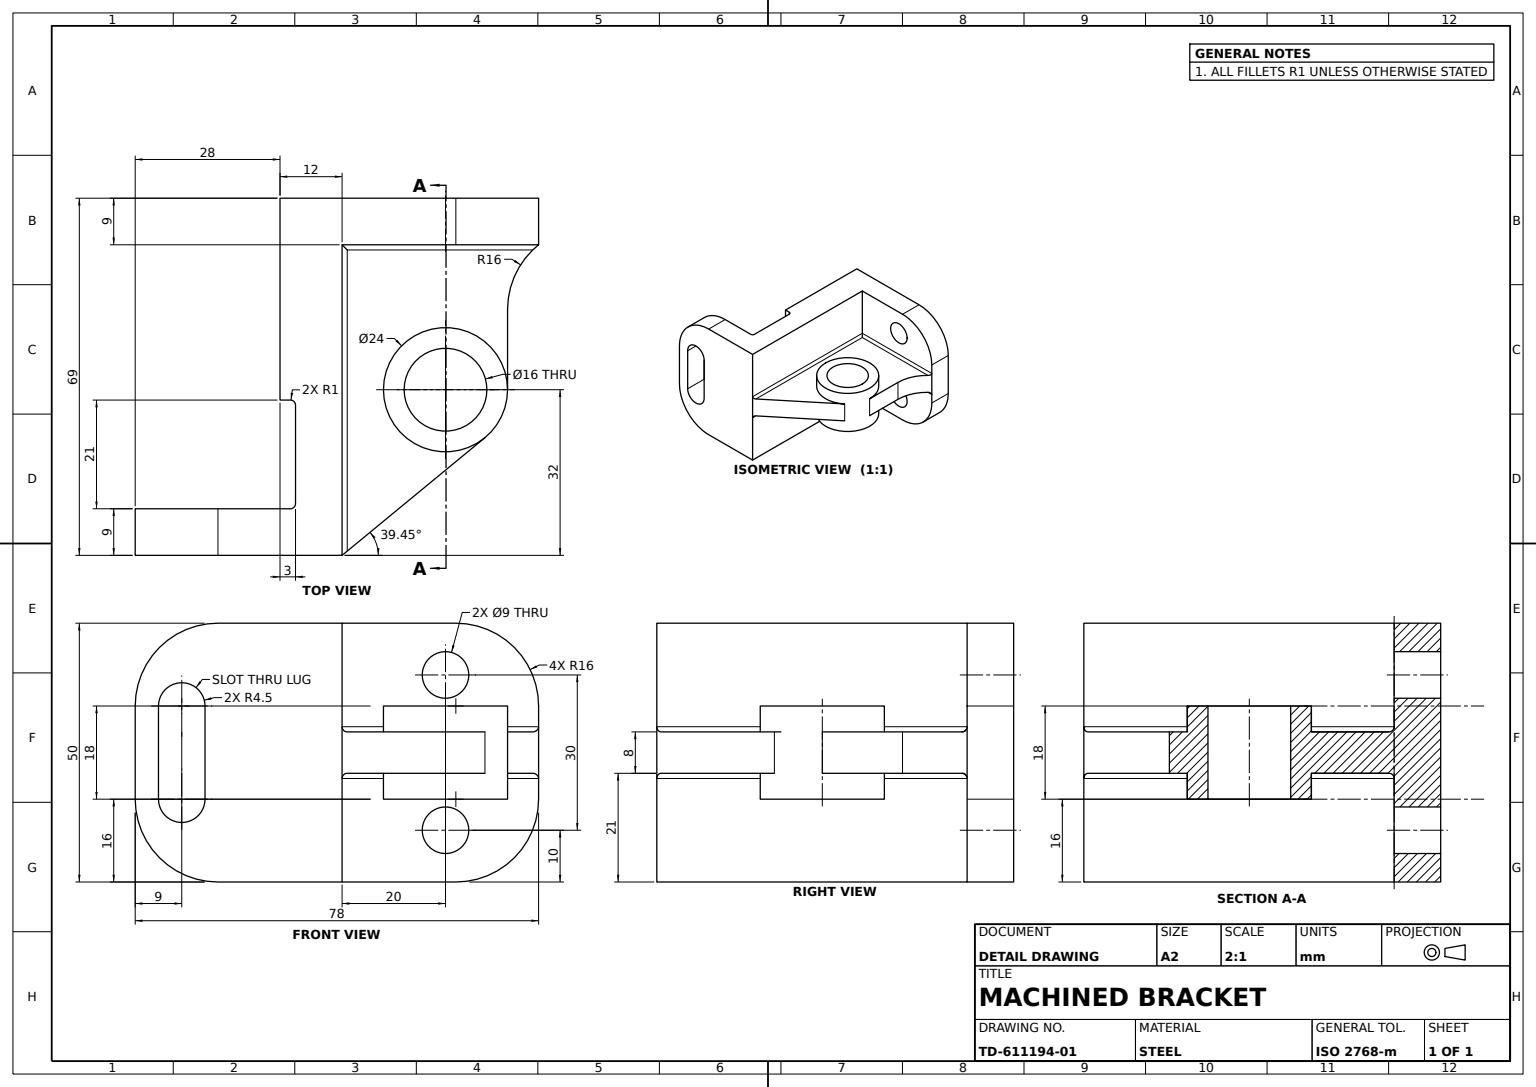
ISO-10303-21;
HEADER;
FILE_DESCRIPTION((''),'2;1');
FILE_NAME('','',(''),(''),'','','');
FILE_SCHEMA(('AUTOMOTIVE_DESIGN'));
ENDSEC;
DATA;
#1=APPLICATION_CONTEXT('');
#2=PRODUCT_CONTEXT('',#1,'mechanical');
#3=PRODUCT('','','',(#2));
#4=PRODUCT_DEFINITION_FORMATION('','',#3);
#5=PRODUCT_DEFINITION_CONTEXT('',#1,'design');
#6=PRODUCT_DEFINITION('','',#4,#5);
#7=PRODUCT_DEFINITION_SHAPE('','',#6);
#8=(LENGTH_UNIT()NAMED_UNIT(*)SI_UNIT(.MILLI.,.METRE.));
#9=(NAMED_UNIT(*)PLANE_ANGLE_UNIT()SI_UNIT($,.RADIAN.));
#10=(NAMED_UNIT(*)SI_UNIT($,.STERADIAN.)SOLID_ANGLE_UNIT());
#11=UNCERTAINTY_MEASURE_WITH_UNIT(LENGTH_MEASURE(1.E-05),#8,'distance_accuracy_value','');
#12=(GEOMETRIC_REPRESENTATION_CONTEXT(3)GLOBAL_UNCERTAINTY_ASSIGNED_CONTEXT((#11))GLOBAL_UNIT_ASSIGNED_CONTEXT((#8,#9,#10))REPRESENTATION_CONTEXT('',''));
#13=CARTESIAN_POINT('',(11.765801,-4.,-27.625282));
#14=VERTEX_POINT('',#13);
#15=CARTESIAN_POINT('',(33.677051,-4.,-1.));
#16=VERTEX_POINT('',#15);
#17=CARTESIAN_POINT('',(34.500404,-4.,0.000491));
#18=DIRECTION('',(0.635440172,0.,0.772150107));
#19=VECTOR('',#18,1000.);
#20=LINE('',#17,#19);
#21=EDGE_CURVE('',#14,#16,#20,.T.);
#22=ORIENTED_EDGE('',*,*,#21,.F.);
#23=CARTESIAN_POINT('',(11.765801,4.,-27.625282));
#24=VERTEX_POINT('',#23);
#25=CARTESIAN_POINT('',(11.765801,-14.,-27.625282));
#26=DIRECTION('',(0.,1.,0.));
#27=VECTOR('',#26,1000.);
#28=LINE('',#25,#27);
#29=EDGE_CURVE('',#14,#24,#28,.T.);
#30=ORIENTED_EDGE('',*,*,#29,.T.);
#31=CARTESIAN_POINT('',(33.677051,4.,-1.));
#32=VERTEX_POINT('',#31);
#33=CARTESIAN_POINT('',(34.5,4.,0.));
#34=LINE('',#33,#19);
#35=EDGE_CURVE('',#24,#32,#34,.T.);
#36=ORIENTED_EDGE('',*,*,#35,.T.);
#37=CARTESIAN_POINT('',(34.5,5.,0.));
#38=VERTEX_POINT('',#37);
#39=CARTESIAN_POINT('',(34.159123,4.,-0.414214));
#40=CARTESIAN_POINT('',(34.5,4.414214,0.));
#41=(BOUNDED_CURVE()B_SPLINE_CURVE(3,(#31,#39,#40,#37),.UNSPECIFIED.,.F.,.T.)B_SPLINE_CURVE_WITH_KNOTS((4,4),(1.570796327,3.141592654),.UNSPECIFIED.)CURVE()GEOMETRIC_REPRESENTATION_ITEM()RATIONAL_B_SPLINE_CURVE((1.,0.804737854,0.804737854,1.))REPRESENTATION_ITEM(''));
#42=EDGE_CURVE('',#32,#38,#41,.T.);
#43=ORIENTED_EDGE('',*,*,#42,.T.);
#44=CARTESIAN_POINT('',(34.5,-5.,0.));
#45=VERTEX_POINT('',#44);
#46=CARTESIAN_POINT('',(34.5,-25.,0.));
#47=DIRECTION('',(0.,-1.,0.));
#48=VECTOR('',#47,1000.);
#49=LINE('',#46,#48);
#50=EDGE_CURVE('',#38,#45,#49,.T.);
#51=ORIENTED_EDGE('',*,*,#50,.T.);
#52=CARTESIAN_POINT('',(34.5,-4.414214,0.));
#53=CARTESIAN_POINT('',(34.159123,-4.,-0.414214));
#54=(BOUNDED_CURVE()B_SPLINE_CURVE(3,(#44,#52,#53,#15),.UNSPECIFIED.,.F.,.T.)B_SPLINE_CURVE_WITH_KNOTS((4,4),(3.141592654,4.71238898),.UNSPECIFIED.)CURVE()GEOMETRIC_REPRESENTATION_ITEM()RATIONAL_B_SPLINE_CURVE((1.,0.804737854,0.804737854,1.))REPRESENTATION_ITEM(''));
#55=EDGE_CURVE('',#45,#16,#54,.T.);
#56=ORIENTED_EDGE('',*,*,#55,.T.);
#57=EDGE_LOOP('',(#22,#30,#36,#43,#51,#56));
#58=FACE_OUTER_BOUND('',#57,.T.);
#59=CARTESIAN_POINT('',(34.5,-14.,0.));
#60=DIRECTION('',(-0.772150107,0.,0.635440172));
#61=AXIS2_PLACEMENT_3D('',#59,#60,#18);
#62=PLANE('',#61);
#63=ADVANCED_FACE('',(#58),#62,.F.);
#64=CARTESIAN_POINT('',(-25.5,-5.,0.));
#65=VERTEX_POINT('',#64);
#66=CARTESIAN_POINT('',(-24.5,-4.,-1.));
#67=VERTEX_POINT('',#66);
#68=CARTESIAN_POINT('',(-25.5,-4.414214,0.));
#69=CARTESIAN_POINT('',(-25.085786,-4.,-0.414214));
#70=(BOUNDED_CURVE()B_SPLINE_CURVE(3,(#64,#68,#69,#66),.UNSPECIFIED.,.F.,.T.)B_SPLINE_CURVE_WITH_KNOTS((4,4),(0.,1.570796327),.UNSPECIFIED.)CURVE()GEOMETRIC_REPRESENTATION_ITEM()RATIONAL_B_SPLINE_CURVE((1.,0.804737854,0.804737854,1.))REPRESENTATION_ITEM(''));
#71=EDGE_CURVE('',#65,#67,#70,.T.);
#72=ORIENTED_EDGE('',*,*,#71,.F.);
#73=CARTESIAN_POINT('',(-25.5,-5.,-38.));
#74=VERTEX_POINT('',#73);
#75=CARTESIAN_POINT('',(-25.5,-5.,-1.));
#76=DIRECTION('',(0.,0.,1.));
#77=VECTOR('',#76,1000.);
#78=LINE('',#75,#77);
#79=EDGE_CURVE('',#74,#65,#78,.T.);
#80=ORIENTED_EDGE('',*,*,#79,.F.);
#81=CARTESIAN_POINT('',(-24.5,-4.,-36.86537));
#82=VERTEX_POINT('',#81);
#83=CARTESIAN_POINT('',(-24.61585,-4.,-36.984917));
#84=CARTESIAN_POINT('',(-24.727494,-4.019528,-37.103853));
#85=CARTESIAN_POINT('',(-24.942978,-4.096203,-37.340276));
#86=CARTESIAN_POINT('',(-25.047494,-4.154192,-37.458663));
#87=CARTESIAN_POINT('',(-25.236204,-4.312145,-37.678131));
#88=CARTESIAN_POINT('',(-25.323005,-4.413693,-37.78232));
#89=CARTESIAN_POINT('',(-25.455791,-4.672041,-37.944486));
#90=CARTESIAN_POINT('',(-25.5,-4.83192,-38.));
#91=B_SPLINE_CURVE_WITH_KNOTS('',3,(#81,#83,#84,#85,#86,#87,#88,#89,#90,#73),.UNSPECIFIED.,.F.,.F.,(4,2,2,2,4),(0.,0.000492283,0.000984567,0.00147685,0.001969133),.UNSPECIFIED.);
#92=EDGE_CURVE('',#82,#74,#91,.T.);
#93=ORIENTED_EDGE('',*,*,#92,.F.);
#94=CARTESIAN_POINT('',(-24.5,-4.,-38.));
#95=DIRECTION('',(0.,0.,-1.));
#96=VECTOR('',#95,1000.);
#97=LINE('',#94,#96);
#98=EDGE_CURVE('',#67,#82,#97,.T.);
#99=ORIENTED_EDGE('',*,*,#98,.F.);
#100=EDGE_LOOP('',(#72,#80,#93,#99));
#101=FACE_OUTER_BOUND('',#100,.T.);
#102=CARTESIAN_POINT('',(-24.5,-5.,0.));
#103=DIRECTION('',(1.,0.,0.));
#104=AXIS2_PLACEMENT_3D('',#102,#76,#103);
#105=CYLINDRICAL_SURFACE('',#104,1.);
#106=ADVANCED_FACE('',(#101),#105,.F.);
#107=CARTESIAN_POINT('',(-25.5,-25.,0.));
#108=VERTEX_POINT('',#107);
#109=CARTESIAN_POINT('',(-25.5,25.,0.));
#110=LINE('',#109,#48);
#111=EDGE_CURVE('',#65,#108,#110,.T.);
#112=ORIENTED_EDGE('',*,*,#111,.F.);
#113=CARTESIAN_POINT('',(0.,-5.,0.));
#114=VECTOR('',#103,1000.);
#115=LINE('',#113,#114);
#116=EDGE_CURVE('',#65,#45,#115,.T.);
#117=ORIENTED_EDGE('',*,*,#116,.T.);
#118=VERTEX_POINT('',#46);
#119=LINE('',#46,#27);
#120=EDGE_CURVE('',#118,#45,#119,.T.);
#121=ORIENTED_EDGE('',*,*,#120,.F.);
#122=CARTESIAN_POINT('',(-34.5,-25.,0.));
#123=LINE('',#122,#114);
#124=EDGE_CURVE('',#108,#118,#123,.T.);
#125=ORIENTED_EDGE('',*,*,#124,.F.);
#126=EDGE_LOOP('',(#112,#117,#121,#125));
#127=FACE_OUTER_BOUND('',#126,.T.);
#128=CARTESIAN_POINT('',(0.,0.,0.));
#129=DIRECTION('',(-1.,0.,0.));
#130=AXIS2_PLACEMENT_3D('',#128,#95,#129);
#131=PLANE('',#130);
#132=ADVANCED_FACE('',(#127),#131,.T.);
#133=CARTESIAN_POINT('',(25.5,25.,24.));
#134=VERTEX_POINT('',#133);
#135=CARTESIAN_POINT('',(25.5,25.,10.));
#136=VERTEX_POINT('',#135);
#137=CARTESIAN_POINT('',(25.5,25.,12.));
#138=LINE('',#137,#96);
#139=EDGE_CURVE('',#134,#136,#138,.T.);
#140=ORIENTED_EDGE('',*,*,#139,.F.);
#141=CARTESIAN_POINT('',(34.5,25.,24.));
#142=VERTEX_POINT('',#141);
#143=LINE('',#141,#114);
#144=EDGE_CURVE('',#134,#142,#143,.T.);
#145=ORIENTED_EDGE('',*,*,#144,.T.);
#146=CARTESIAN_POINT('',(34.5,25.,0.));
#147=VERTEX_POINT('',#146);
#148=CARTESIAN_POINT('',(34.5,25.,12.));
#149=LINE('',#148,#96);
#150=EDGE_CURVE('',#142,#147,#149,.T.);
#151=ORIENTED_EDGE('',*,*,#150,.T.);
#152=VERTEX_POINT('',#109);
#153=CARTESIAN_POINT('',(-34.5,25.,0.));
#154=VECTOR('',#129,1000.);
#155=LINE('',#153,#154);
#156=EDGE_CURVE('',#147,#152,#155,.T.);
#157=ORIENTED_EDGE('',*,*,#156,.T.);
#158=CARTESIAN_POINT('',(-25.5,25.,-22.));
#159=VERTEX_POINT('',#158);
#160=CARTESIAN_POINT('',(-25.5,25.,-38.));
#161=LINE('',#160,#77);
#162=EDGE_CURVE('',#159,#152,#161,.T.);
#163=ORIENTED_EDGE('',*,*,#162,.F.);
#164=CARTESIAN_POINT('',(-34.5,25.,-22.));
#165=VERTEX_POINT('',#164);
#166=LINE('',#164,#154);
#167=EDGE_CURVE('',#159,#165,#166,.T.);
#168=ORIENTED_EDGE('',*,*,#167,.T.);
#169=CARTESIAN_POINT('',(-34.5,25.,12.));
#170=VERTEX_POINT('',#169);
#171=LINE('',#169,#96);
#172=EDGE_CURVE('',#170,#165,#171,.T.);
#173=ORIENTED_EDGE('',*,*,#172,.F.);
#174=CARTESIAN_POINT('',(4.5,25.,12.));
#175=VERTEX_POINT('',#174);
#176=LINE('',#169,#154);
#177=EDGE_CURVE('',#175,#170,#176,.T.);
#178=ORIENTED_EDGE('',*,*,#177,.F.);
#179=CARTESIAN_POINT('',(4.5,25.,10.));
#180=VERTEX_POINT('',#179);
#181=LINE('',#174,#77);
#182=EDGE_CURVE('',#180,#175,#181,.T.);
#183=ORIENTED_EDGE('',*,*,#182,.F.);
#184=CARTESIAN_POINT('',(5.5,25.,9.));
#185=VERTEX_POINT('',#184);
#186=CARTESIAN_POINT('',(5.5,25.,10.));
#187=AXIS2_PLACEMENT_3D('',#186,#47,#95);
#188=CIRCLE('',#187,1.);
#189=EDGE_CURVE('',#180,#185,#188,.T.);
#190=ORIENTED_EDGE('',*,*,#189,.T.);
#191=CARTESIAN_POINT('',(24.5,25.,9.));
#192=VERTEX_POINT('',#191);
#193=CARTESIAN_POINT('',(4.5,25.,9.));
#194=LINE('',#193,#154);
#195=EDGE_CURVE('',#192,#185,#194,.T.);
#196=ORIENTED_EDGE('',*,*,#195,.F.);
#197=CARTESIAN_POINT('',(24.5,25.,10.));
#198=AXIS2_PLACEMENT_3D('',#197,#47,#95);
#199=CIRCLE('',#198,1.);
#200=EDGE_CURVE('',#192,#136,#199,.T.);
#201=ORIENTED_EDGE('',*,*,#200,.T.);
#202=EDGE_LOOP('',(#140,#145,#151,#157,#163,#168,#173,#178,#183,#190,#196,#201));
#203=FACE_OUTER_BOUND('',#202,.T.);
#204=AXIS2_PLACEMENT_3D('',#169,#47,#95);
#205=PLANE('',#204);
#206=ADVANCED_FACE('',(#203),#205,.F.);
#207=CARTESIAN_POINT('',(-34.5,-15.,-24.5));
#208=VERTEX_POINT('',#207);
#209=CARTESIAN_POINT('',(-34.5,-15.,-15.5));
#210=VERTEX_POINT('',#209);
#211=CARTESIAN_POINT('',(-34.5,-15.,-20.));
#212=AXIS2_PLACEMENT_3D('',#211,#129,#76);
#213=CIRCLE('',#212,4.5);
#214=EDGE_CURVE('',#208,#210,#213,.T.);
#215=ORIENTED_EDGE('',*,*,#214,.T.);
#216=CARTESIAN_POINT('',(-25.5,-15.,-15.5));
#217=VERTEX_POINT('',#216);
#218=CARTESIAN_POINT('',(3.5,-15.,-15.5));
#219=LINE('',#218,#154);
#220=EDGE_CURVE('',#217,#210,#219,.T.);
#221=ORIENTED_EDGE('',*,*,#220,.F.);
#222=CARTESIAN_POINT('',(-25.5,-15.,-24.5));
#223=VERTEX_POINT('',#222);
#224=CARTESIAN_POINT('',(-25.5,-15.,-20.));
#225=AXIS2_PLACEMENT_3D('',#224,#129,#47);
#226=CIRCLE('',#225,4.5);
#227=EDGE_CURVE('',#223,#217,#226,.T.);
#228=ORIENTED_EDGE('',*,*,#227,.F.);
#229=CARTESIAN_POINT('',(3.5,-15.,-24.5));
#230=LINE('',#229,#154);
#231=EDGE_CURVE('',#223,#208,#230,.T.);
#232=ORIENTED_EDGE('',*,*,#231,.T.);
#233=EDGE_LOOP('',(#215,#221,#228,#232));
#234=FACE_OUTER_BOUND('',#233,.T.);
#235=CARTESIAN_POINT('',(3.5,-15.,-20.));
#236=AXIS2_PLACEMENT_3D('',#235,#129,#76);
#237=CYLINDRICAL_SURFACE('',#236,4.5);
#238=ADVANCED_FACE('',(#234),#237,.F.);
#239=CARTESIAN_POINT('',(34.5,-9.,40.));
#240=VERTEX_POINT('',#239);
#241=CARTESIAN_POINT('',(34.5,9.,40.));
#242=VERTEX_POINT('',#241);
#243=CARTESIAN_POINT('',(34.5,-25.,40.));
#244=LINE('',#243,#27);
#245=EDGE_CURVE('',#240,#242,#244,.T.);
#246=ORIENTED_EDGE('',*,*,#245,.T.);
#247=CARTESIAN_POINT('',(25.5,9.,40.));
#248=VERTEX_POINT('',#247);
#249=LINE('',#247,#154);
#250=EDGE_CURVE('',#242,#248,#249,.T.);
#251=ORIENTED_EDGE('',*,*,#250,.T.);
#252=CARTESIAN_POINT('',(25.5,-9.,40.));
#253=VERTEX_POINT('',#252);
#254=CARTESIAN_POINT('',(25.5,25.,40.));
#255=LINE('',#254,#48);
#256=EDGE_CURVE('',#248,#253,#255,.T.);
#257=ORIENTED_EDGE('',*,*,#256,.T.);
#258=LINE('',#239,#114);
#259=EDGE_CURVE('',#253,#240,#258,.T.);
#260=ORIENTED_EDGE('',*,*,#259,.T.);
#261=EDGE_LOOP('',(#246,#251,#257,#260));
#262=FACE_OUTER_BOUND('',#261,.T.);
#263=CARTESIAN_POINT('',(0.,0.,40.));
#264=AXIS2_PLACEMENT_3D('',#263,#76,#103);
#265=PLANE('',#264);
#266=ADVANCED_FACE('',(#262),#265,.T.);
#267=CARTESIAN_POINT('',(-34.5,9.,-38.));
#268=VERTEX_POINT('',#267);
#269=CARTESIAN_POINT('',(-25.5,9.,-38.));
#270=VERTEX_POINT('',#269);
#271=CARTESIAN_POINT('',(0.,9.,-38.));
#272=LINE('',#271,#114);
#273=EDGE_CURVE('',#268,#270,#272,.T.);
#274=ORIENTED_EDGE('',*,*,#273,.F.);
#275=CARTESIAN_POINT('',(-34.5,9.,-22.));
#276=AXIS2_PLACEMENT_3D('',#275,#129,#95);
#277=CIRCLE('',#276,16.);
#278=EDGE_CURVE('',#165,#268,#277,.T.);
#279=ORIENTED_EDGE('',*,*,#278,.F.);
#280=ORIENTED_EDGE('',*,*,#167,.F.);
#281=CARTESIAN_POINT('',(-25.5,9.,-22.));
#282=AXIS2_PLACEMENT_3D('',#281,#103,#47);
#283=CIRCLE('',#282,16.);
#284=EDGE_CURVE('',#270,#159,#283,.T.);
#285=ORIENTED_EDGE('',*,*,#284,.F.);
#286=EDGE_LOOP('',(#274,#279,#280,#285));
#287=FACE_OUTER_BOUND('',#286,.T.);
#288=CARTESIAN_POINT('',(0.,9.,-22.));
#289=AXIS2_PLACEMENT_3D('',#288,#103,#95);
#290=CYLINDRICAL_SURFACE('',#289,16.);
#291=ADVANCED_FACE('',(#287),#290,.T.);
#292=CARTESIAN_POINT('',(2.5,9.,-8.));
#293=VERTEX_POINT('',#292);
#294=CARTESIAN_POINT('',(2.5,4.,-8.));
#295=VERTEX_POINT('',#294);
#296=LINE('',#292,#48);
#297=EDGE_CURVE('',#293,#295,#296,.T.);
#298=ORIENTED_EDGE('',*,*,#297,.F.);
#299=CARTESIAN_POINT('',(2.5,9.,-32.));
#300=VERTEX_POINT('',#299);
#301=CARTESIAN_POINT('',(2.5,9.,-20.));
#302=AXIS2_PLACEMENT_3D('',#301,#26,#76);
#303=CIRCLE('',#302,12.);
#304=EDGE_CURVE('',#300,#293,#303,.T.);
#305=ORIENTED_EDGE('',*,*,#304,.F.);
#306=CARTESIAN_POINT('',(2.5,4.,-32.));
#307=VERTEX_POINT('',#306);
#308=LINE('',#299,#48);
#309=EDGE_CURVE('',#300,#307,#308,.T.);
#310=ORIENTED_EDGE('',*,*,#309,.T.);
#311=CARTESIAN_POINT('',(2.5,4.,-20.));
#312=AXIS2_PLACEMENT_3D('',#311,#26,#103);
#313=CIRCLE('',#312,12.);
#314=EDGE_CURVE('',#307,#295,#313,.T.);
#315=ORIENTED_EDGE('',*,*,#314,.T.);
#316=EDGE_LOOP('',(#298,#305,#310,#315));
#317=FACE_OUTER_BOUND('',#316,.T.);
#318=AXIS2_PLACEMENT_3D('',#301,#47,#95);
#319=CYLINDRICAL_SURFACE('',#318,12.);
#320=ADVANCED_FACE('',(#317),#319,.T.);
#321=CARTESIAN_POINT('',(2.5,-9.,-32.));
#322=VERTEX_POINT('',#321);
#323=CARTESIAN_POINT('',(2.5,-9.,-8.));
#324=VERTEX_POINT('',#323);
#325=CARTESIAN_POINT('',(2.5,-9.,-20.));
#326=AXIS2_PLACEMENT_3D('',#325,#26,#76);
#327=CIRCLE('',#326,12.);
#328=EDGE_CURVE('',#322,#324,#327,.T.);
#329=ORIENTED_EDGE('',*,*,#328,.T.);
#330=CARTESIAN_POINT('',(2.5,-4.,-8.));
#331=VERTEX_POINT('',#330);
#332=EDGE_CURVE('',#331,#324,#296,.T.);
#333=ORIENTED_EDGE('',*,*,#332,.F.);
#334=CARTESIAN_POINT('',(2.5,-4.,-32.));
#335=VERTEX_POINT('',#334);
#336=CARTESIAN_POINT('',(2.5,-4.,-20.));
#337=AXIS2_PLACEMENT_3D('',#336,#47,#129);
#338=CIRCLE('',#337,12.);
#339=EDGE_CURVE('',#331,#335,#338,.T.);
#340=ORIENTED_EDGE('',*,*,#339,.T.);
#341=EDGE_CURVE('',#335,#322,#308,.T.);
#342=ORIENTED_EDGE('',*,*,#341,.T.);
#343=EDGE_LOOP('',(#329,#333,#340,#342));
#344=FACE_OUTER_BOUND('',#343,.T.);
#345=ADVANCED_FACE('',(#344),#319,.T.);
#346=CARTESIAN_POINT('',(-34.5,-25.,12.));
#347=VERTEX_POINT('',#346);
#348=LINE('',#346,#48);
#349=EDGE_CURVE('',#170,#347,#348,.T.);
#350=ORIENTED_EDGE('',*,*,#349,.T.);
#351=CARTESIAN_POINT('',(4.5,-25.,12.));
#352=VERTEX_POINT('',#351);
#353=LINE('',#346,#114);
#354=EDGE_CURVE('',#347,#352,#353,.T.);
#355=ORIENTED_EDGE('',*,*,#354,.T.);
#356=LINE('',#351,#27);
#357=EDGE_CURVE('',#352,#175,#356,.T.);
#358=ORIENTED_EDGE('',*,*,#357,.T.);
#359=ORIENTED_EDGE('',*,*,#177,.T.);
#360=EDGE_LOOP('',(#350,#355,#358,#359));
#361=FACE_OUTER_BOUND('',#360,.T.);
#362=CARTESIAN_POINT('',(0.,0.,12.));
#363=AXIS2_PLACEMENT_3D('',#362,#95,#129);
#364=PLANE('',#363);
#365=ADVANCED_FACE('',(#361),#364,.F.);
#366=CARTESIAN_POINT('',(-34.5,-25.,-22.));
#367=VERTEX_POINT('',#366);
#368=LINE('',#346,#96);
#369=EDGE_CURVE('',#347,#367,#368,.T.);
#370=ORIENTED_EDGE('',*,*,#369,.T.);
#371=CARTESIAN_POINT('',(-25.5,-25.,-22.));
#372=VERTEX_POINT('',#371);
#373=LINE('',#366,#114);
#374=EDGE_CURVE('',#367,#372,#373,.T.);
#375=ORIENTED_EDGE('',*,*,#374,.T.);
#376=CARTESIAN_POINT('',(-25.5,-25.,-38.));
#377=LINE('',#376,#77);
#378=EDGE_CURVE('',#372,#108,#377,.T.);
#379=ORIENTED_EDGE('',*,*,#378,.T.);
#380=ORIENTED_EDGE('',*,*,#124,.T.);
#381=CARTESIAN_POINT('',(34.5,-25.,24.));
#382=VERTEX_POINT('',#381);
#383=CARTESIAN_POINT('',(34.5,-25.,12.));
#384=LINE('',#383,#96);
#385=EDGE_CURVE('',#382,#118,#384,.T.);
#386=ORIENTED_EDGE('',*,*,#385,.F.);
#387=CARTESIAN_POINT('',(25.5,-25.,24.));
#388=VERTEX_POINT('',#387);
#389=LINE('',#387,#154);
#390=EDGE_CURVE('',#382,#388,#389,.T.);
#391=ORIENTED_EDGE('',*,*,#390,.T.);
#392=CARTESIAN_POINT('',(25.5,-25.,10.));
#393=VERTEX_POINT('',#392);
#394=CARTESIAN_POINT('',(25.5,-25.,12.));
#395=LINE('',#394,#96);
#396=EDGE_CURVE('',#388,#393,#395,.T.);
#397=ORIENTED_EDGE('',*,*,#396,.T.);
#398=CARTESIAN_POINT('',(24.5,-25.,9.));
#399=VERTEX_POINT('',#398);
#400=CARTESIAN_POINT('',(24.5,-25.,10.));
#401=AXIS2_PLACEMENT_3D('',#400,#26,#76);
#402=CIRCLE('',#401,1.);
#403=EDGE_CURVE('',#393,#399,#402,.T.);
#404=ORIENTED_EDGE('',*,*,#403,.T.);
#405=CARTESIAN_POINT('',(5.5,-25.,9.));
#406=VERTEX_POINT('',#405);
#407=CARTESIAN_POINT('',(4.5,-25.,9.));
#408=LINE('',#407,#154);
#409=EDGE_CURVE('',#399,#406,#408,.T.);
#410=ORIENTED_EDGE('',*,*,#409,.T.);
#411=CARTESIAN_POINT('',(4.5,-25.,10.));
#412=VERTEX_POINT('',#411);
#413=CARTESIAN_POINT('',(5.5,-25.,10.));
#414=AXIS2_PLACEMENT_3D('',#413,#26,#76);
#415=CIRCLE('',#414,1.);
#416=EDGE_CURVE('',#406,#412,#415,.T.);
#417=ORIENTED_EDGE('',*,*,#416,.T.);
#418=LINE('',#351,#77);
#419=EDGE_CURVE('',#412,#352,#418,.T.);
#420=ORIENTED_EDGE('',*,*,#419,.T.);
#421=ORIENTED_EDGE('',*,*,#354,.F.);
#422=EDGE_LOOP('',(#370,#375,#379,#380,#386,#391,#397,#404,#410,#417,#420,#421));
#423=FACE_OUTER_BOUND('',#422,.T.);
#424=AXIS2_PLACEMENT_3D('',#346,#26,#76);
#425=PLANE('',#424);
#426=ADVANCED_FACE('',(#423),#425,.F.);
#427=ORIENTED_EDGE('',*,*,#231,.F.);
#428=EDGE_CURVE('',#217,#223,#226,.T.);
#429=ORIENTED_EDGE('',*,*,#428,.F.);
#430=ORIENTED_EDGE('',*,*,#220,.T.);
#431=EDGE_CURVE('',#210,#208,#213,.T.);
#432=ORIENTED_EDGE('',*,*,#431,.T.);
#433=EDGE_LOOP('',(#427,#429,#430,#432));
#434=FACE_OUTER_BOUND('',#433,.T.);
#435=ADVANCED_FACE('',(#434),#237,.F.);
#436=EDGE_CURVE('',#295,#24,#313,.T.);
#437=ORIENTED_EDGE('',*,*,#436,.T.);
#438=ORIENTED_EDGE('',*,*,#29,.F.);
#439=EDGE_CURVE('',#14,#331,#338,.T.);
#440=ORIENTED_EDGE('',*,*,#439,.T.);
#441=ORIENTED_EDGE('',*,*,#332,.T.);
#442=EDGE_CURVE('',#324,#322,#327,.T.);
#443=ORIENTED_EDGE('',*,*,#442,.T.);
#444=ORIENTED_EDGE('',*,*,#341,.F.);
#445=CARTESIAN_POINT('',(2.5,-14.,-32.));
#446=LINE('',#445,#27);
#447=EDGE_CURVE('',#335,#307,#446,.T.);
#448=ORIENTED_EDGE('',*,*,#447,.T.);
#449=ORIENTED_EDGE('',*,*,#309,.F.);
#450=EDGE_CURVE('',#293,#300,#303,.T.);
#451=ORIENTED_EDGE('',*,*,#450,.F.);
#452=ORIENTED_EDGE('',*,*,#297,.T.);
#453=EDGE_LOOP('',(#437,#438,#440,#441,#443,#444,#448,#449,#451,#452));
#454=FACE_OUTER_BOUND('',#453,.T.);
#455=ADVANCED_FACE('',(#454),#319,.T.);
#456=CARTESIAN_POINT('',(25.5,9.,26.5));
#457=VERTEX_POINT('',#456);
#458=CARTESIAN_POINT('',(25.5,9.,35.5));
#459=VERTEX_POINT('',#458);
#460=CARTESIAN_POINT('',(25.5,9.,31.));
#461=AXIS2_PLACEMENT_3D('',#460,#103,#95);
#462=CIRCLE('',#461,4.5);
#463=EDGE_CURVE('',#457,#459,#462,.T.);
#464=ORIENTED_EDGE('',*,*,#463,.F.);
#465=CARTESIAN_POINT('',(34.5,9.,26.5));
#466=VERTEX_POINT('',#465);
#467=CARTESIAN_POINT('',(6.5,9.,26.5));
#468=LINE('',#467,#114);
#469=EDGE_CURVE('',#457,#466,#468,.T.);
#470=ORIENTED_EDGE('',*,*,#469,.T.);
#471=CARTESIAN_POINT('',(34.5,9.,35.5));
#472=VERTEX_POINT('',#471);
#473=CARTESIAN_POINT('',(34.5,9.,31.));
#474=AXIS2_PLACEMENT_3D('',#473,#103,#95);
#475=CIRCLE('',#474,4.5);
#476=EDGE_CURVE('',#466,#472,#475,.T.);
#477=ORIENTED_EDGE('',*,*,#476,.T.);
#478=CARTESIAN_POINT('',(6.5,9.,35.5));
#479=LINE('',#478,#114);
#480=EDGE_CURVE('',#459,#472,#479,.T.);
#481=ORIENTED_EDGE('',*,*,#480,.F.);
#482=EDGE_LOOP('',(#464,#470,#477,#481));
#483=FACE_OUTER_BOUND('',#482,.T.);
#484=CARTESIAN_POINT('',(6.5,9.,31.));
#485=AXIS2_PLACEMENT_3D('',#484,#103,#95);
#486=CYLINDRICAL_SURFACE('',#485,4.5);
#487=ADVANCED_FACE('',(#483),#486,.F.);
#488=CARTESIAN_POINT('',(34.501,-4.,-1.));
#489=LINE('',#488,#154);
#490=EDGE_CURVE('',#16,#67,#489,.T.);
#491=ORIENTED_EDGE('',*,*,#490,.T.);
#492=ORIENTED_EDGE('',*,*,#98,.T.);
#493=CARTESIAN_POINT('',(-13.010004,-4.,-32.));
#494=VERTEX_POINT('',#493);
#495=CARTESIAN_POINT('',(-13.010004,-4.,-48.));
#496=AXIS2_PLACEMENT_3D('',#495,#26,#129);
#497=CIRCLE('',#496,16.);
#498=EDGE_CURVE('',#82,#494,#497,.T.);
#499=ORIENTED_EDGE('',*,*,#498,.T.);
#500=CARTESIAN_POINT('',(34.501,-4.,-32.));
#501=LINE('',#500,#114);
#502=EDGE_CURVE('',#494,#335,#501,.T.);
#503=ORIENTED_EDGE('',*,*,#502,.T.);
#504=ORIENTED_EDGE('',*,*,#339,.F.);
#505=ORIENTED_EDGE('',*,*,#439,.F.);
#506=ORIENTED_EDGE('',*,*,#21,.T.);
#507=EDGE_LOOP('',(#491,#492,#499,#503,#504,#505,#506));
#508=FACE_OUTER_BOUND('',#507,.T.);
#509=CARTESIAN_POINT('',(34.501,-4.,0.));
#510=AXIS2_PLACEMENT_3D('',#509,#26,#129);
#511=PLANE('',#510);
#512=ADVANCED_FACE('',(#508),#511,.F.);
#513=CARTESIAN_POINT('',(-25.5,15.,-15.5));
#514=VERTEX_POINT('',#513);
#515=CARTESIAN_POINT('',(-34.5,15.,-15.5));
#516=VERTEX_POINT('',#515);
#517=CARTESIAN_POINT('',(3.5,15.,-15.5));
#518=LINE('',#517,#154);
#519=EDGE_CURVE('',#514,#516,#518,.T.);
#520=ORIENTED_EDGE('',*,*,#519,.F.);
#521=CARTESIAN_POINT('',(-25.5,15.,-24.5));
#522=VERTEX_POINT('',#521);
#523=CARTESIAN_POINT('',(-25.5,15.,-20.));
#524=AXIS2_PLACEMENT_3D('',#523,#129,#47);
#525=CIRCLE('',#524,4.5);
#526=EDGE_CURVE('',#522,#514,#525,.T.);
#527=ORIENTED_EDGE('',*,*,#526,.F.);
#528=CARTESIAN_POINT('',(-34.5,15.,-24.5));
#529=VERTEX_POINT('',#528);
#530=CARTESIAN_POINT('',(3.5,15.,-24.5));
#531=LINE('',#530,#154);
#532=EDGE_CURVE('',#522,#529,#531,.T.);
#533=ORIENTED_EDGE('',*,*,#532,.T.);
#534=CARTESIAN_POINT('',(-34.5,15.,-20.));
#535=AXIS2_PLACEMENT_3D('',#534,#129,#76);
#536=CIRCLE('',#535,4.5);
#537=EDGE_CURVE('',#529,#516,#536,.T.);
#538=ORIENTED_EDGE('',*,*,#537,.T.);
#539=EDGE_LOOP('',(#520,#527,#533,#538));
#540=FACE_OUTER_BOUND('',#539,.T.);
#541=CARTESIAN_POINT('',(3.5,15.,-20.));
#542=AXIS2_PLACEMENT_3D('',#541,#129,#76);
#543=CYLINDRICAL_SURFACE('',#542,4.5);
#544=ADVANCED_FACE('',(#540),#543,.F.);
#545=EDGE_CURVE('',#514,#522,#525,.T.);
#546=ORIENTED_EDGE('',*,*,#545,.T.);
#547=ORIENTED_EDGE('',*,*,#526,.T.);
#548=EDGE_LOOP('',(#546,#547));
#549=FACE_BOUND('',#548,.T.);
#550=CARTESIAN_POINT('',(-25.5,5.,0.));
#551=VERTEX_POINT('',#550);
#552=CARTESIAN_POINT('',(-25.5,5.,-38.));
#553=VERTEX_POINT('',#552);
#554=LINE('',#552,#96);
#555=EDGE_CURVE('',#551,#553,#554,.T.);
#556=ORIENTED_EDGE('',*,*,#555,.T.);
#557=LINE('',#160,#48);
#558=EDGE_CURVE('',#270,#553,#557,.T.);
#559=ORIENTED_EDGE('',*,*,#558,.F.);
#560=ORIENTED_EDGE('',*,*,#284,.T.);
#561=ORIENTED_EDGE('',*,*,#162,.T.);
#562=EDGE_CURVE('',#152,#551,#110,.T.);
#563=ORIENTED_EDGE('',*,*,#562,.T.);
#564=EDGE_LOOP('',(#556,#559,#560,#561,#563));
#565=FACE_OUTER_BOUND('',#564,.T.);
#566=AXIS2_PLACEMENT_3D('',#160,#129,#47);
#567=PLANE('',#566);
#568=ADVANCED_FACE('',(#549,#565),#567,.F.);
#569=CARTESIAN_POINT('',(-24.5,4.,-1.));
#570=VERTEX_POINT('',#569);
#571=CARTESIAN_POINT('',(-25.085786,4.,-0.414214));
#572=CARTESIAN_POINT('',(-25.5,4.414214,0.));
#573=(BOUNDED_CURVE()B_SPLINE_CURVE(3,(#569,#571,#572,#550),.UNSPECIFIED.,.F.,.T.)B_SPLINE_CURVE_WITH_KNOTS((4,4),(1.570796327,3.141592654),.UNSPECIFIED.)CURVE()GEOMETRIC_REPRESENTATION_ITEM()RATIONAL_B_SPLINE_CURVE((1.,0.804737854,0.804737854,1.))REPRESENTATION_ITEM(''));
#574=EDGE_CURVE('',#570,#551,#573,.T.);
#575=ORIENTED_EDGE('',*,*,#574,.F.);
#576=CARTESIAN_POINT('',(-24.5,4.,-36.86537));
#577=VERTEX_POINT('',#576);
#578=LINE('',#569,#77);
#579=EDGE_CURVE('',#577,#570,#578,.T.);
#580=ORIENTED_EDGE('',*,*,#579,.F.);
#581=CARTESIAN_POINT('',(-25.5,4.831875,-38.));
#582=CARTESIAN_POINT('',(-25.456556,4.673863,-37.945428));
#583=CARTESIAN_POINT('',(-25.32319,4.41372,-37.782538));
#584=CARTESIAN_POINT('',(-25.237078,4.313022,-37.679163));
#585=CARTESIAN_POINT('',(-25.047988,4.154463,-37.459224));
#586=CARTESIAN_POINT('',(-24.945591,4.097336,-37.343178));
#587=CARTESIAN_POINT('',(-24.727975,4.0195,-37.104347));
#588=CARTESIAN_POINT('',(-24.61577,4.,-36.984835));
#589=B_SPLINE_CURVE_WITH_KNOTS('',3,(#552,#581,#582,#583,#584,#585,#586,#587,#588,#576),.UNSPECIFIED.,.F.,.F.,(4,2,2,2,4),(0.,0.000494621,0.000989242,0.001483863,0.001978485),.UNSPECIFIED.);
#590=EDGE_CURVE('',#553,#577,#589,.T.);
#591=ORIENTED_EDGE('',*,*,#590,.F.);
#592=ORIENTED_EDGE('',*,*,#555,.F.);
#593=EDGE_LOOP('',(#575,#580,#591,#592));
#594=FACE_OUTER_BOUND('',#593,.T.);
#595=CARTESIAN_POINT('',(-24.5,5.,0.));
#596=AXIS2_PLACEMENT_3D('',#595,#95,#129);
#597=CYLINDRICAL_SURFACE('',#596,1.);
#598=ADVANCED_FACE('',(#594),#597,.F.);
#599=CARTESIAN_POINT('',(0.,5.,0.));
#600=LINE('',#599,#154);
#601=EDGE_CURVE('',#38,#551,#600,.T.);
#602=ORIENTED_EDGE('',*,*,#601,.T.);
#603=ORIENTED_EDGE('',*,*,#562,.F.);
#604=ORIENTED_EDGE('',*,*,#156,.F.);
#605=EDGE_CURVE('',#38,#147,#119,.T.);
#606=ORIENTED_EDGE('',*,*,#605,.F.);
#607=EDGE_LOOP('',(#602,#603,#604,#606));
#608=FACE_OUTER_BOUND('',#607,.T.);
#609=ADVANCED_FACE('',(#608),#131,.T.);
#610=LINE('',#405,#48);
#611=EDGE_CURVE('',#185,#406,#610,.T.);
#612=ORIENTED_EDGE('',*,*,#611,.F.);
#613=ORIENTED_EDGE('',*,*,#189,.F.);
#614=LINE('',#179,#27);
#615=EDGE_CURVE('',#412,#180,#614,.T.);
#616=ORIENTED_EDGE('',*,*,#615,.F.);
#617=ORIENTED_EDGE('',*,*,#416,.F.);
#618=EDGE_LOOP('',(#612,#613,#616,#617));
#619=FACE_OUTER_BOUND('',#618,.T.);
#620=AXIS2_PLACEMENT_3D('',#413,#47,#95);
#621=CYLINDRICAL_SURFACE('',#620,1.);
#622=ADVANCED_FACE('',(#619),#621,.F.);
#623=CARTESIAN_POINT('',(-13.010004,4.,-32.));
#624=VERTEX_POINT('',#623);
#625=CARTESIAN_POINT('',(-13.010004,4.,-48.));
#626=AXIS2_PLACEMENT_3D('',#625,#47,#103);
#627=CIRCLE('',#626,16.);
#628=EDGE_CURVE('',#624,#577,#627,.T.);
#629=ORIENTED_EDGE('',*,*,#628,.T.);
#630=ORIENTED_EDGE('',*,*,#579,.T.);
#631=CARTESIAN_POINT('',(34.501,4.,-1.));
#632=LINE('',#631,#114);
#633=EDGE_CURVE('',#570,#32,#632,.T.);
#634=ORIENTED_EDGE('',*,*,#633,.T.);
#635=ORIENTED_EDGE('',*,*,#35,.F.);
#636=ORIENTED_EDGE('',*,*,#436,.F.);
#637=ORIENTED_EDGE('',*,*,#314,.F.);
#638=LINE('',#306,#114);
#639=EDGE_CURVE('',#624,#307,#638,.T.);
#640=ORIENTED_EDGE('',*,*,#639,.F.);
#641=EDGE_LOOP('',(#629,#630,#634,#635,#636,#637,#640));
#642=FACE_OUTER_BOUND('',#641,.T.);
#643=CARTESIAN_POINT('',(34.501,4.,0.));
#644=AXIS2_PLACEMENT_3D('',#643,#47,#103);
#645=PLANE('',#644);
#646=ADVANCED_FACE('',(#642),#645,.F.);
#647=ORIENTED_EDGE('',*,*,#403,.F.);
#648=LINE('',#392,#48);
#649=EDGE_CURVE('',#136,#393,#648,.T.);
#650=ORIENTED_EDGE('',*,*,#649,.F.);
#651=ORIENTED_EDGE('',*,*,#200,.F.);
#652=LINE('',#191,#27);
#653=EDGE_CURVE('',#399,#192,#652,.T.);
#654=ORIENTED_EDGE('',*,*,#653,.F.);
#655=EDGE_LOOP('',(#647,#650,#651,#654));
#656=FACE_OUTER_BOUND('',#655,.T.);
#657=AXIS2_PLACEMENT_3D('',#400,#47,#95);
#658=CYLINDRICAL_SURFACE('',#657,1.);
#659=ADVANCED_FACE('',(#656),#658,.F.);
#660=ORIENTED_EDGE('',*,*,#195,.T.);
#661=ORIENTED_EDGE('',*,*,#611,.T.);
#662=ORIENTED_EDGE('',*,*,#409,.F.);
#663=ORIENTED_EDGE('',*,*,#653,.T.);
#664=EDGE_LOOP('',(#660,#661,#662,#663));
#665=FACE_OUTER_BOUND('',#664,.T.);
#666=AXIS2_PLACEMENT_3D('',#407,#95,#129);
#667=PLANE('',#666);
#668=ADVANCED_FACE('',(#665),#667,.F.);
#669=ORIENTED_EDGE('',*,*,#639,.T.);
#670=ORIENTED_EDGE('',*,*,#447,.F.);
#671=ORIENTED_EDGE('',*,*,#502,.F.);
#672=CARTESIAN_POINT('',(-13.010004,-14.,-32.));
#673=LINE('',#672,#27);
#674=EDGE_CURVE('',#494,#624,#673,.T.);
#675=ORIENTED_EDGE('',*,*,#674,.T.);
#676=EDGE_LOOP('',(#669,#670,#671,#675));
#677=FACE_OUTER_BOUND('',#676,.T.);
#678=AXIS2_PLACEMENT_3D('',#445,#76,#103);
#679=PLANE('',#678);
#680=ADVANCED_FACE('',(#677),#679,.F.);
#681=ORIENTED_EDGE('',*,*,#144,.F.);
#682=CARTESIAN_POINT('',(25.5,9.,24.));
#683=AXIS2_PLACEMENT_3D('',#682,#129,#95);
#684=CIRCLE('',#683,16.);
#685=EDGE_CURVE('',#248,#134,#684,.T.);
#686=ORIENTED_EDGE('',*,*,#685,.F.);
#687=ORIENTED_EDGE('',*,*,#250,.F.);
#688=CARTESIAN_POINT('',(34.5,9.,24.));
#689=AXIS2_PLACEMENT_3D('',#688,#103,#76);
#690=CIRCLE('',#689,16.);
#691=EDGE_CURVE('',#142,#242,#690,.T.);
#692=ORIENTED_EDGE('',*,*,#691,.F.);
#693=EDGE_LOOP('',(#681,#686,#687,#692));
#694=FACE_OUTER_BOUND('',#693,.T.);
#695=CARTESIAN_POINT('',(0.,9.,24.));
#696=AXIS2_PLACEMENT_3D('',#695,#103,#95);
#697=CYLINDRICAL_SURFACE('',#696,16.);
#698=ADVANCED_FACE('',(#694),#697,.T.);
#699=EDGE_CURVE('',#516,#529,#536,.T.);
#700=ORIENTED_EDGE('',*,*,#699,.F.);
#701=ORIENTED_EDGE('',*,*,#537,.F.);
#702=EDGE_LOOP('',(#700,#701));
#703=FACE_BOUND('',#702,.T.);
#704=ORIENTED_EDGE('',*,*,#431,.F.);
#705=ORIENTED_EDGE('',*,*,#214,.F.);
#706=EDGE_LOOP('',(#704,#705));
#707=FACE_BOUND('',#706,.T.);
#708=ORIENTED_EDGE('',*,*,#369,.F.);
#709=ORIENTED_EDGE('',*,*,#349,.F.);
#710=ORIENTED_EDGE('',*,*,#172,.T.);
#711=ORIENTED_EDGE('',*,*,#278,.T.);
#712=CARTESIAN_POINT('',(-34.5,-9.,-38.));
#713=VERTEX_POINT('',#712);
#714=CARTESIAN_POINT('',(-34.5,25.,-38.));
#715=LINE('',#714,#27);
#716=EDGE_CURVE('',#713,#268,#715,.T.);
#717=ORIENTED_EDGE('',*,*,#716,.F.);
#718=CARTESIAN_POINT('',(-34.5,-9.,-22.));
#719=AXIS2_PLACEMENT_3D('',#718,#129,#95);
#720=CIRCLE('',#719,16.);
#721=EDGE_CURVE('',#713,#367,#720,.T.);
#722=ORIENTED_EDGE('',*,*,#721,.T.);
#723=EDGE_LOOP('',(#708,#709,#710,#711,#717,#722));
#724=FACE_OUTER_BOUND('',#723,.T.);
#725=AXIS2_PLACEMENT_3D('',#346,#103,#95);
#726=PLANE('',#725);
#727=ADVANCED_FACE('',(#703,#707,#724),#726,.F.);
#728=ORIENTED_EDGE('',*,*,#532,.F.);
#729=ORIENTED_EDGE('',*,*,#545,.F.);
#730=ORIENTED_EDGE('',*,*,#519,.T.);
#731=ORIENTED_EDGE('',*,*,#699,.T.);
#732=EDGE_LOOP('',(#728,#729,#730,#731));
#733=FACE_OUTER_BOUND('',#732,.T.);
#734=ADVANCED_FACE('',(#733),#543,.F.);
#735=CARTESIAN_POINT('',(2.5,9.,-28.));
#736=VERTEX_POINT('',#735);
#737=CARTESIAN_POINT('',(2.5,9.,-12.));
#738=VERTEX_POINT('',#737);
#739=CIRCLE('',#302,8.);
#740=EDGE_CURVE('',#736,#738,#739,.T.);
#741=ORIENTED_EDGE('',*,*,#740,.F.);
#742=EDGE_CURVE('',#738,#736,#739,.T.);
#743=ORIENTED_EDGE('',*,*,#742,.F.);
#744=EDGE_LOOP('',(#741,#743));
#745=FACE_BOUND('',#744,.T.);
#746=ORIENTED_EDGE('',*,*,#450,.T.);
#747=ORIENTED_EDGE('',*,*,#304,.T.);
#748=EDGE_LOOP('',(#746,#747));
#749=FACE_OUTER_BOUND('',#748,.T.);
#750=PLANE('',#302);
#751=ADVANCED_FACE('',(#745,#749),#750,.T.);
#752=CARTESIAN_POINT('',(2.5,-9.,-28.));
#753=VERTEX_POINT('',#752);
#754=CARTESIAN_POINT('',(2.5,-9.,-12.));
#755=VERTEX_POINT('',#754);
#756=CIRCLE('',#326,8.);
#757=EDGE_CURVE('',#753,#755,#756,.T.);
#758=ORIENTED_EDGE('',*,*,#757,.T.);
#759=EDGE_CURVE('',#755,#753,#756,.T.);
#760=ORIENTED_EDGE('',*,*,#759,.T.);
#761=EDGE_LOOP('',(#758,#760));
#762=FACE_BOUND('',#761,.T.);
#763=ORIENTED_EDGE('',*,*,#442,.F.);
#764=ORIENTED_EDGE('',*,*,#328,.F.);
#765=EDGE_LOOP('',(#763,#764));
#766=FACE_OUTER_BOUND('',#765,.T.);
#767=PLANE('',#326);
#768=ADVANCED_FACE('',(#762,#766),#767,.F.);
#769=ORIENTED_EDGE('',*,*,#227,.T.);
#770=ORIENTED_EDGE('',*,*,#428,.T.);
#771=EDGE_LOOP('',(#769,#770));
#772=FACE_BOUND('',#771,.T.);
#773=ORIENTED_EDGE('',*,*,#378,.F.);
#774=CARTESIAN_POINT('',(-25.5,-9.,-38.));
#775=VERTEX_POINT('',#774);
#776=CARTESIAN_POINT('',(-25.5,-9.,-22.));
#777=AXIS2_PLACEMENT_3D('',#776,#103,#47);
#778=CIRCLE('',#777,16.);
#779=EDGE_CURVE('',#372,#775,#778,.T.);
#780=ORIENTED_EDGE('',*,*,#779,.T.);
#781=EDGE_CURVE('',#74,#775,#557,.T.);
#782=ORIENTED_EDGE('',*,*,#781,.F.);
#783=ORIENTED_EDGE('',*,*,#79,.T.);
#784=ORIENTED_EDGE('',*,*,#111,.T.);
#785=EDGE_LOOP('',(#773,#780,#782,#783,#784));
#786=FACE_OUTER_BOUND('',#785,.T.);
#787=ADVANCED_FACE('',(#772,#786),#567,.F.);
#788=ORIENTED_EDGE('',*,*,#182,.T.);
#789=ORIENTED_EDGE('',*,*,#357,.F.);
#790=ORIENTED_EDGE('',*,*,#419,.F.);
#791=ORIENTED_EDGE('',*,*,#615,.T.);
#792=EDGE_LOOP('',(#788,#789,#790,#791));
#793=FACE_OUTER_BOUND('',#792,.T.);
#794=AXIS2_PLACEMENT_3D('',#351,#129,#76);
#795=PLANE('',#794);
#796=ADVANCED_FACE('',(#793),#795,.F.);
#797=ORIENTED_EDGE('',*,*,#628,.F.);
#798=ORIENTED_EDGE('',*,*,#674,.F.);
#799=ORIENTED_EDGE('',*,*,#498,.F.);
#800=ORIENTED_EDGE('',*,*,#92,.T.);
#801=EDGE_CURVE('',#553,#74,#557,.T.);
#802=ORIENTED_EDGE('',*,*,#801,.F.);
#803=ORIENTED_EDGE('',*,*,#590,.T.);
#804=EDGE_LOOP('',(#797,#798,#799,#800,#802,#803));
#805=FACE_OUTER_BOUND('',#804,.T.);
#806=CARTESIAN_POINT('',(-13.010004,25.,-48.));
#807=AXIS2_PLACEMENT_3D('',#806,#26,#129);
#808=CYLINDRICAL_SURFACE('',#807,16.);
#809=ADVANCED_FACE('',(#805),#808,.F.);
#810=ORIENTED_EDGE('',*,*,#42,.F.);
#811=ORIENTED_EDGE('',*,*,#633,.F.);
#812=ORIENTED_EDGE('',*,*,#574,.T.);
#813=ORIENTED_EDGE('',*,*,#601,.F.);
#814=EDGE_LOOP('',(#810,#811,#812,#813));
#815=FACE_OUTER_BOUND('',#814,.T.);
#816=CARTESIAN_POINT('',(0.,5.,-1.));
#817=AXIS2_PLACEMENT_3D('',#816,#129,#47);
#818=CYLINDRICAL_SURFACE('',#817,1.);
#819=ADVANCED_FACE('',(#815),#818,.F.);
#820=ORIENTED_EDGE('',*,*,#779,.F.);
#821=ORIENTED_EDGE('',*,*,#374,.F.);
#822=ORIENTED_EDGE('',*,*,#721,.F.);
#823=CARTESIAN_POINT('',(0.,-9.,-38.));
#824=LINE('',#823,#154);
#825=EDGE_CURVE('',#775,#713,#824,.T.);
#826=ORIENTED_EDGE('',*,*,#825,.F.);
#827=EDGE_LOOP('',(#820,#821,#822,#826));
#828=FACE_OUTER_BOUND('',#827,.T.);
#829=CARTESIAN_POINT('',(0.,-9.,-22.));
#830=AXIS2_PLACEMENT_3D('',#829,#129,#76);
#831=CYLINDRICAL_SURFACE('',#830,16.);
#832=ADVANCED_FACE('',(#828),#831,.T.);
#833=LINE('',#735,#48);
#834=EDGE_CURVE('',#736,#753,#833,.T.);
#835=ORIENTED_EDGE('',*,*,#834,.F.);
#836=ORIENTED_EDGE('',*,*,#740,.T.);
#837=LINE('',#737,#48);
#838=EDGE_CURVE('',#738,#755,#837,.T.);
#839=ORIENTED_EDGE('',*,*,#838,.T.);
#840=ORIENTED_EDGE('',*,*,#757,.F.);
#841=EDGE_LOOP('',(#835,#836,#839,#840));
#842=FACE_OUTER_BOUND('',#841,.T.);
#843=CYLINDRICAL_SURFACE('',#318,8.);
#844=ADVANCED_FACE('',(#842),#843,.F.);
#845=CARTESIAN_POINT('',(25.5,-9.,26.5));
#846=VERTEX_POINT('',#845);
#847=CARTESIAN_POINT('',(25.5,-25.,26.5));
#848=LINE('',#847,#27);
#849=EDGE_CURVE('',#846,#457,#848,.T.);
#850=ORIENTED_EDGE('',*,*,#849,.T.);
#851=ORIENTED_EDGE('',*,*,#463,.T.);
#852=CARTESIAN_POINT('',(25.5,-9.,35.5));
#853=VERTEX_POINT('',#852);
#854=CARTESIAN_POINT('',(25.5,-25.,35.5));
#855=LINE('',#854,#48);
#856=EDGE_CURVE('',#459,#853,#855,.T.);
#857=ORIENTED_EDGE('',*,*,#856,.T.);
#858=CARTESIAN_POINT('',(25.5,-9.,31.));
#859=AXIS2_PLACEMENT_3D('',#858,#103,#95);
#860=CIRCLE('',#859,4.5);
#861=EDGE_CURVE('',#853,#846,#860,.T.);
#862=ORIENTED_EDGE('',*,*,#861,.T.);
#863=EDGE_LOOP('',(#850,#851,#857,#862));
#864=FACE_BOUND('',#863,.T.);
#865=CARTESIAN_POINT('',(25.5,-9.,24.));
#866=AXIS2_PLACEMENT_3D('',#865,#129,#95);
#867=CIRCLE('',#866,16.);
#868=EDGE_CURVE('',#388,#253,#867,.T.);
#869=ORIENTED_EDGE('',*,*,#868,.T.);
#870=ORIENTED_EDGE('',*,*,#256,.F.);
#871=ORIENTED_EDGE('',*,*,#685,.T.);
#872=ORIENTED_EDGE('',*,*,#139,.T.);
#873=ORIENTED_EDGE('',*,*,#649,.T.);
#874=ORIENTED_EDGE('',*,*,#396,.F.);
#875=EDGE_LOOP('',(#869,#870,#871,#872,#873,#874));
#876=FACE_OUTER_BOUND('',#875,.T.);
#877=AXIS2_PLACEMENT_3D('',#394,#103,#95);
#878=PLANE('',#877);
#879=ADVANCED_FACE('',(#864,#876),#878,.F.);
#880=ORIENTED_EDGE('',*,*,#116,.F.);
#881=ORIENTED_EDGE('',*,*,#71,.T.);
#882=ORIENTED_EDGE('',*,*,#490,.F.);
#883=ORIENTED_EDGE('',*,*,#55,.F.);
#884=EDGE_LOOP('',(#880,#881,#882,#883));
#885=FACE_OUTER_BOUND('',#884,.T.);
#886=CARTESIAN_POINT('',(34.501,-5.,-1.));
#887=AXIS2_PLACEMENT_3D('',#886,#129,#47);
#888=CYLINDRICAL_SURFACE('',#887,1.);
#889=ADVANCED_FACE('',(#885),#888,.F.);
#890=CARTESIAN_POINT('',(34.5,-9.,26.5));
#891=VERTEX_POINT('',#890);
#892=LINE('',#465,#27);
#893=EDGE_CURVE('',#891,#466,#892,.T.);
#894=ORIENTED_EDGE('',*,*,#893,.T.);
#895=ORIENTED_EDGE('',*,*,#469,.F.);
#896=ORIENTED_EDGE('',*,*,#849,.F.);
#897=CARTESIAN_POINT('',(6.5,-9.,26.5));
#898=LINE('',#897,#114);
#899=EDGE_CURVE('',#846,#891,#898,.T.);
#900=ORIENTED_EDGE('',*,*,#899,.T.);
#901=EDGE_LOOP('',(#894,#895,#896,#900));
#902=FACE_OUTER_BOUND('',#901,.T.);
#903=AXIS2_PLACEMENT_3D('',#467,#95,#129);
#904=PLANE('',#903);
#905=ADVANCED_FACE('',(#902),#904,.F.);
#906=CARTESIAN_POINT('',(34.5,-9.,35.5));
#907=VERTEX_POINT('',#906);
#908=CARTESIAN_POINT('',(34.5,-9.,31.));
#909=AXIS2_PLACEMENT_3D('',#908,#103,#95);
#910=CIRCLE('',#909,4.5);
#911=EDGE_CURVE('',#907,#891,#910,.T.);
#912=ORIENTED_EDGE('',*,*,#911,.F.);
#913=LINE('',#471,#48);
#914=EDGE_CURVE('',#472,#907,#913,.T.);
#915=ORIENTED_EDGE('',*,*,#914,.F.);
#916=ORIENTED_EDGE('',*,*,#476,.F.);
#917=ORIENTED_EDGE('',*,*,#893,.F.);
#918=EDGE_LOOP('',(#912,#915,#916,#917));
#919=FACE_BOUND('',#918,.T.);
#920=ORIENTED_EDGE('',*,*,#385,.T.);
#921=ORIENTED_EDGE('',*,*,#120,.T.);
#922=ORIENTED_EDGE('',*,*,#50,.F.);
#923=ORIENTED_EDGE('',*,*,#605,.T.);
#924=ORIENTED_EDGE('',*,*,#150,.F.);
#925=ORIENTED_EDGE('',*,*,#691,.T.);
#926=ORIENTED_EDGE('',*,*,#245,.F.);
#927=CARTESIAN_POINT('',(34.5,-9.,24.));
#928=AXIS2_PLACEMENT_3D('',#927,#103,#76);
#929=CIRCLE('',#928,16.);
#930=EDGE_CURVE('',#240,#382,#929,.T.);
#931=ORIENTED_EDGE('',*,*,#930,.T.);
#932=EDGE_LOOP('',(#920,#921,#922,#923,#924,#925,#926,#931));
#933=FACE_OUTER_BOUND('',#932,.T.);
#934=AXIS2_PLACEMENT_3D('',#383,#129,#76);
#935=PLANE('',#934);
#936=ADVANCED_FACE('',(#919,#933),#935,.F.);
#937=ORIENTED_EDGE('',*,*,#914,.T.);
#938=CARTESIAN_POINT('',(6.5,-9.,35.5));
#939=LINE('',#938,#114);
#940=EDGE_CURVE('',#853,#907,#939,.T.);
#941=ORIENTED_EDGE('',*,*,#940,.F.);
#942=ORIENTED_EDGE('',*,*,#856,.F.);
#943=ORIENTED_EDGE('',*,*,#480,.T.);
#944=EDGE_LOOP('',(#937,#941,#942,#943));
#945=FACE_OUTER_BOUND('',#944,.T.);
#946=AXIS2_PLACEMENT_3D('',#478,#76,#103);
#947=PLANE('',#946);
#948=ADVANCED_FACE('',(#945),#947,.F.);
#949=ORIENTED_EDGE('',*,*,#273,.T.);
#950=ORIENTED_EDGE('',*,*,#558,.T.);
#951=ORIENTED_EDGE('',*,*,#801,.T.);
#952=ORIENTED_EDGE('',*,*,#781,.T.);
#953=ORIENTED_EDGE('',*,*,#825,.T.);
#954=ORIENTED_EDGE('',*,*,#716,.T.);
#955=EDGE_LOOP('',(#949,#950,#951,#952,#953,#954));
#956=FACE_OUTER_BOUND('',#955,.T.);
#957=CARTESIAN_POINT('',(0.,0.,-38.));
#958=AXIS2_PLACEMENT_3D('',#957,#76,#103);
#959=PLANE('',#958);
#960=ADVANCED_FACE('',(#956),#959,.F.);
#961=ORIENTED_EDGE('',*,*,#899,.F.);
#962=ORIENTED_EDGE('',*,*,#861,.F.);
#963=ORIENTED_EDGE('',*,*,#940,.T.);
#964=ORIENTED_EDGE('',*,*,#911,.T.);
#965=EDGE_LOOP('',(#961,#962,#963,#964));
#966=FACE_OUTER_BOUND('',#965,.T.);
#967=CARTESIAN_POINT('',(6.5,-9.,31.));
#968=AXIS2_PLACEMENT_3D('',#967,#103,#95);
#969=CYLINDRICAL_SURFACE('',#968,4.5);
#970=ADVANCED_FACE('',(#966),#969,.F.);
#971=ORIENTED_EDGE('',*,*,#868,.F.);
#972=ORIENTED_EDGE('',*,*,#390,.F.);
#973=ORIENTED_EDGE('',*,*,#930,.F.);
#974=ORIENTED_EDGE('',*,*,#259,.F.);
#975=EDGE_LOOP('',(#971,#972,#973,#974));
#976=FACE_OUTER_BOUND('',#975,.T.);
#977=CARTESIAN_POINT('',(0.,-9.,24.));
#978=AXIS2_PLACEMENT_3D('',#977,#129,#76);
#979=CYLINDRICAL_SURFACE('',#978,16.);
#980=ADVANCED_FACE('',(#976),#979,.T.);
#981=ORIENTED_EDGE('',*,*,#742,.T.);
#982=ORIENTED_EDGE('',*,*,#834,.T.);
#983=ORIENTED_EDGE('',*,*,#759,.F.);
#984=ORIENTED_EDGE('',*,*,#838,.F.);
#985=EDGE_LOOP('',(#981,#982,#983,#984));
#986=FACE_OUTER_BOUND('',#985,.T.);
#987=ADVANCED_FACE('',(#986),#843,.F.);
#988=CLOSED_SHELL('',(#63,#106,#132,#206,#238,#266,#291,#320,#345,#365,#426,#435,#455,#487,#512,#544,#568,#598,#609,#622,#646,#659,#668,#680,#698,#727,#734,#751,#768,#787,#796,#809,#819,#832,#844,#879,#889,#905,#936,#948,#960,#970,#980,#987));
#989=MANIFOLD_SOLID_BREP('',#988);
#990=ADVANCED_BREP_SHAPE_REPRESENTATION('',(#989),#12);
#991=SHAPE_DEFINITION_REPRESENTATION(#7,#990);
ENDSEC;
END-ISO-10303-21;
